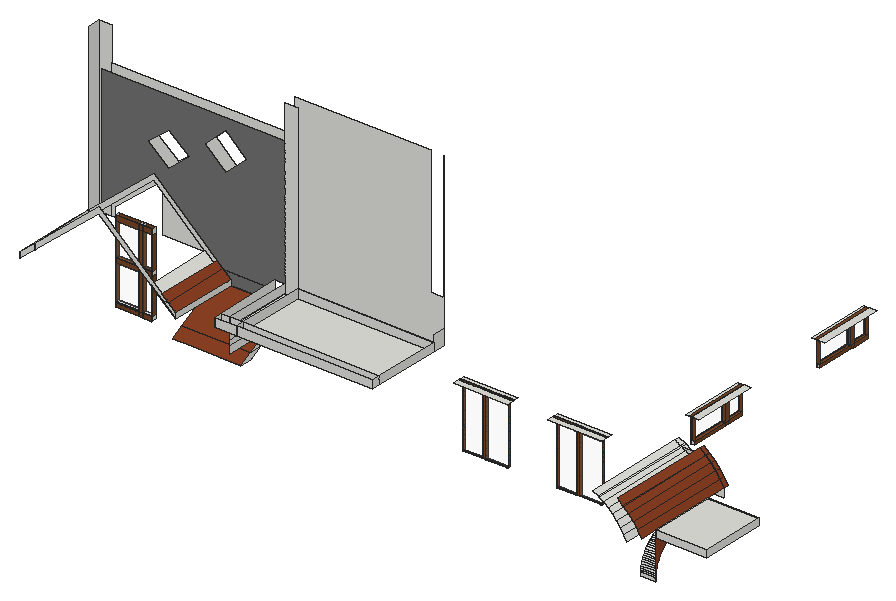
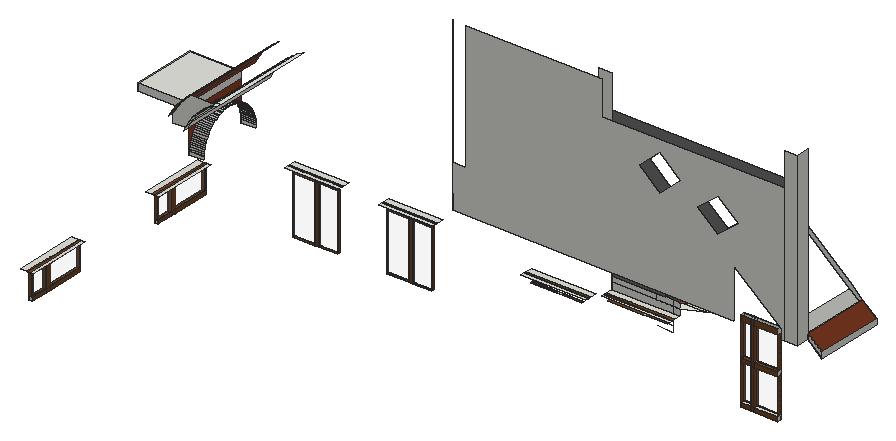
# SketchUp Ruby script. Lengths in inches.
U = 1.inch
M = Sketchup.active_model
def pt(a) = Geom::Point3d.new(a.map { |v| v * U })
def face(e, loops, mat)
  f = e.add_face(loops[0].map { |a| pt(a) })
  loops[1..].each { |l| e.add_face(l.map { |a| pt(a) }).erase! }
  f.material = f.back_material = mat if mat
  f
end
# faces: each face lists its corners as indices into pts; further lists are holes
def faces(e, pts, list, mat = nil) = list.each { |f| face(e, (f[0].is_a?(Array) ? f : [f]).map { |l| l.map { |i| pts[i] } }, mat) }
# xy, xz, yz: faces in a plane at the given z, y or x. An outline is a flat list of corners, or four numbers for a rectangle; further outlines are holes
def ring(l) = l.size == 4 ? [[l[0], l[1]], [l[2], l[1]], [l[2], l[3]], [l[0], l[3]]] : l.each_slice(2).to_a
def flat(e, list, mat, &to3) = list.each { |f| face(e, (f[0].is_a?(Array) ? f : [f]).map { |l| ring(l).map { |u, v| to3.(u, v) } }, mat) }
def xy(e, z, list, mat = nil) = flat(e, list, mat) { |x, y| [x, y, z] }
def xz(e, y, list, mat = nil) = flat(e, list, mat) { |x, z| [x, y, z] }
def yz(e, x, list, mat = nil) = flat(e, list, mat) { |y, z| [x, y, z] }
def lines(e, pts, list) = list.each { |a, b| e.add_line(pt(pts[a]), pt(pts[b])) }
# prism: a flat outline (further loops are holes) pulled along v
def prism(e, loops, v, mat = nil)
  f = face(e, loops, mat); d = Geom::Vector3d.new(v.map { |x| x * U })
  f.pushpull(f.normal.samedirection?(d) ? d.length : -d.length)
end
def box(e, o, s, mat = nil) = prism(e, [[o, [o[0] + s[0], o[1], o[2]], [o[0] + s[0], o[1] + s[1], o[2]], [o[0], o[1] + s[1], o[2]]]], [0, 0, s[2]], mat)
def at(x, y, z, deg = 0) = Geom::Transformation.translation(pt([x, y, z])) * Geom::Transformation.rotation(ORIGIN, Z_AXIS, deg.degrees)
def axes(o, x, y, z) = Geom::Transformation.new([*x, 0, *y, 0, *z, 0, *pt(o).to_a, 1])
def part(name) = M.definitions.add(name)
# library, detail: a bought-in or finely detailed component or shape, given as its bounding box
def library(name, o, s) = part(name).tap { |d| box(d.entities, o, s) }
def detail(e, o, s) = box(e.add_group.entities, o, s)
def put(e, d, t, mat = nil) = e.add_instance(d, t).tap { |i| i.material = mat if mat }
def group(e, t, mat = nil) = e.add_group.tap { |g| g.transformation = t; g.material = mat if mat }.entities
root = M.entities
M.materials.add("Glass Thin Clear 001").color = [243, 240, 240]
M.materials["Glass Thin Clear 001"].alpha = 0.1
M.materials.add("[Color M05]").color = [114, 114, 114]
M.materials.add("[Roofing Tile Spanish]").color = [138, 64, 36]
M.materials.add("[Wood Veneer 01]").color = [120, 70, 37]
xy(root,61.76,[[283.58,170.5625,285.96,172.1875],[349.83,170.5625,352.21,172.1875]])
xy(root,61.76,[[270.03,170.5625,283.58,170.875],[285.96,170.5625,301.89,170.875],[336.28,170.5625,349.83,170.875],[352.21,170.5625,368.14,170.875],[270.03,170.875,283.58,172.1875],
  [285.96,170.875,301.89,172.1875],[336.28,170.875,349.83,172.1875],[352.21,170.875,368.14,172.1875]],"[Wood Veneer 01]")
xy(root,66.22,[[41.61,170.5625,44.06,171.0625],[41.61,171.0625,44.06,173.875]])
xy(root,66.22,[[25.1,170.5625,41.61,171.0625],[44.06,170.5625,50.73,171.0625],[25.1,171.0625,41.61,173.875],[44.06,171.0625,50.73,173.875]],"[Wood Veneer 01]")
xy(root,69.18,[[41.61,170.5625,44.06,171.0625],[25.1,171.0625,41.61,173.875],[41.61,171.0625,44.06,173.875],[44.06,171.0625,50.73,173.875]])
xy(root,69.18,[[25.1,170.5625,41.61,171.0625],[44.06,170.5625,50.73,171.0625]],"[Wood Veneer 01]")
xy(root,91.5625,[[99.96,127.4375,99.96,135.72,113.85,135.72,113.21,127.4375],[113.21,127.4375,113.85,135.72,147.96,135.72,147.96,127.4375]])
xy(root,91.75,[[177.76,170.5625,182.03,172.375]])
xy(root,91.75,[[163.76,170.5625,177.76,170.875],[182.03,170.5625,200.3125,170.875],[163.76,170.875,177.76,172.375],[182.03,170.875,200.3125,172.375]],"[Wood Veneer 01]")
xy(root,93.98,[[399.27,210.14,401.46,237.2],[398.84,237.2,401.46,239.92],[399.27,239.92,401.46,252.12],[399.27,320.77,401.46,347.83],[398.84,347.83,401.46,350.54],
  [399.27,350.54,401.46,362.74]])
xy(root,93.98,[[398.84,210.14,399.27,237.2],[398.84,239.92,399.27,252.12],[398.84,320.77,399.27,347.83],[398.84,350.54,399.27,362.74]],"[Wood Veneer 01]")
xy(root,94.5,[[41.61,170.5625,44.06,171.0625],[41.61,171.0625,44.06,173.875]])
xy(root,94.5,[[25.1,170.5625,41.61,171.0625],[44.06,170.5625,50.73,171.0625],[25.1,171.0625,41.61,173.875],[44.06,171.0625,50.73,173.875]],"[Wood Veneer 01]")
xy(root,95.875,[[99.96,135.72,101.32,135.72,101.9375,143.8,99.96,143.8],[101.32,135.72,113.85,135.72,114.47,143.8,101.9375,143.8],[113.85,135.72,147.96,135.72,147.96,143.8,114.47,143.8]])
xy(root,96.1,[[159.41,166.0625,204.66,170.5625],[159.41,172.375,204.66,175.0625]])
xy(root,96.1,[[159.41,170.5625,204.66,171.8125],[159.41,171.8125,204.66,172.375]],"[Wood Veneer 01]")
xy(root,96.26,[[398.84,237.2,401.46,239.92],[398.84,347.83,401.46,350.54]])
xy(root,96.26,[[398.84,210.14,399.27,237.2],[399.27,210.14,401.46,237.2],[398.84,239.92,399.27,252.12],[399.27,239.92,401.46,252.12],[398.84,320.77,399.27,347.83],
  [399.27,320.77,401.46,347.83],[398.84,350.54,399.27,362.74],[399.27,350.54,401.46,362.74]],"[Wood Veneer 01]")
xy(root,97.27,[[25.1,170.5625,41.61,171.0625],[41.61,170.5625,44.06,171.0625],[44.06,170.5625,50.73,171.0625],[41.61,171.0625,44.06,173.875]])
xy(root,97.27,[[25.1,171.0625,41.61,173.875],[44.06,171.0625,50.73,173.875]],"[Wood Veneer 01]")
xy(root,100.14,[[117.68,170.5625,120.35,173.4375]])
xy(root,100.14,[[102.81,170.5625,117.68,171.125],[120.35,170.5625,145.12,171.125],[102.81,171.125,117.68,173.4375],[120.35,171.125,145.12,173.4375]],"[Wood Veneer 01]")
xy(root,100.61,[[457.27,105.875,493.27,151.74]])
xy(root,101.99,[[283.58,170.5625,285.96,172.1875],[349.83,170.5625,352.21,172.1875]])
xy(root,101.99,[[270.03,170.5625,283.58,170.875],[285.96,170.5625,301.89,170.875],[336.28,170.5625,349.83,170.875],[352.21,170.5625,368.14,170.875],[270.03,170.875,283.58,172.1875],
  [285.96,170.875,301.89,172.1875],[336.28,170.875,349.83,172.1875],[352.21,170.875,368.14,172.1875]],"[Wood Veneer 01]")
xy(root,102.98,[[99.96,166.0625,147.96,170.5625],[99.96,173.4375,147.96,175.0625]])
xy(root,102.98,[[99.96,170.5625,147.96,172.375],[99.96,172.375,147.96,173.4375]],"[Wood Veneer 01]")
xy(root,105.09,[[266.93,166.0625,304.99,170.5625],[333.18,166.0625,371.24,170.5625],[266.93,172.1875,304.99,175.0625],[333.18,172.1875,371.24,175.0625]])
xy(root,105.09,[[266.93,170.5625,304.99,171.8125],[333.18,170.5625,371.24,171.8125],[266.93,171.8125,304.99,172.1875],[333.18,171.8125,371.24,172.1875]],"[Wood Veneer 01]")
xy(root,105.64,[[457.27,105.875,493.27,151.74]])
xy(root,110.75,[[399.27,210.14,401.46,237.2],[398.84,237.2,401.46,239.92],[399.27,239.92,401.46,252.12],[399.27,320.77,401.46,347.83],[398.84,347.83,401.46,350.54],
  [399.27,350.54,401.46,362.74]])
xy(root,110.75,[[398.84,210.14,399.27,237.2],[398.84,239.92,399.27,252.12],[398.84,320.77,399.27,347.83],[398.84,350.54,399.27,362.74]],"[Wood Veneer 01]")
xy(root,112.57,[[396.96,208.32,398.84,253.94],[401.46,208.32,405.96,253.94],[396.96,318.94,398.84,364.57],[401.46,318.94,405.96,364.57]])
xy(root,112.57,[[398.84,208.32,400.59,253.94],[400.59,208.32,401.46,253.94],[398.84,318.94,400.59,364.57],[400.59,318.94,401.46,364.57]],"[Wood Veneer 01]")
xy(root,120,[[141.15,112.5625,156.96,118.0625],[156.96,112.5625,252.96,118.0625],[99.96,118.0625,99.96,166.0625,103.65,166.0625,100.75,128.39,104.53,128.1,104.53,118.0625],[141.15,118.0625,147.96,166.0625],[147.96,118.0625,156.96,166.0625],
  [156.96,118.0625,252.96,166.0625],[104.53,128.1,100.75,128.39,103.65,166.0625,104.53,166.0625],[103.65,166.0625,116.18,166.0625,103.72,167.02]])
xy(root,120.79,[[41.61,170.5625,44.06,171.0625],[41.61,171.0625,44.06,173.875]])
xy(root,120.79,[[25.1,170.5625,41.61,171.0625],[44.06,170.5625,50.73,171.0625],[25.1,171.0625,41.61,173.875],[44.06,171.0625,50.73,173.875]],"[Wood Veneer 01]")
xz(root,105.875,[[446.88,73.29,457.27,75.69],[457.27,100.61,493.27,105.64]])
xz(root,112.5625,[[141.15,120,156.96,126],[156.96,120,252.96,126]])
xz(root,118.0625,[[0,111.45,9.96,120,9.96,124,0,115.45],[109.72,111.45,109.72,115.45,104.53,120,99.96,120],[9.96,120,18.96,127.72,55.42,159,91.87,127.08,99.96,120,104.53,120,99.96,124,55.42,163,18.96,131.72,9.96,124],[141.15,120,147.96,126],[147.96,120,156.96,126],
  [156.96,120,252.96,126]])
xz(root,151.74,[[446.88,73.29,457.27,75.69],[446.88,75.69,457.27,75.78],[457.27,100.61,493.27,105.64]])
xz(root,166.0625,[[446.88,99.6875,457.27,99.6875,457.27,105.64,454.61,110.13,451.55,114.36,448.11,118.29,444.67,121.5625,427.48,121.5625,430.54,119.68,434.02,117.06,437.24,114.11,440.16,110.87,442.75,107.36,445,103.62],[99.96,102.98,147.96,107.76],[99.96,107.76,99.96,111.67,109.47,111.67,109.72,111.45,109.72,111.67,116.18,111.67,116.18,107.76],[116.18,107.76,147.96,111.67],[0,111.45,0,115.45,9.96,124,9.96,120],
  [109.72,111.45,109.47,111.67,109.72,111.67],[109.47,111.67,99.96,120,104.53,120,109.72,115.45,109.72,111.67],[9.96,120,9.96,124,18.96,131.72,55.42,163,99.96,124,104.53,120,99.96,120,91.87,127.08,55.42,159,18.96,127.72],[147.96,120,156.96,240],[156.96,120,252.96,126]])
xz(root,166.0625,[[99.96,111.67,109.47,111.67,99.96,120],[109.72,111.67,147.96,111.67,147.96,120,104.53,120,109.72,115.45],[[104.53,120,141.15,120,141.15,126,147.96,126,147.96,216.17,18.96,216.17,18.96,131.72,55.42,163,99.96,124],[106.65,181.57,91.87,195.01,106.65,208.45,121.43,195.01],[66.04,170.09,51.29,182.43,66.04,194.78,80.79,182.43]]],"[Color M05]")
xz(root,170.5625,[[283.58,61.76,285.96,101.99],[349.83,61.76,352.21,101.99],[25.1,66.22,41.61,69.18],[41.61,66.22,44.06,69.18],[44.06,66.22,50.73,69.18],
  [41.61,69.18,44.06,94.5],[25.1,94.5,41.61,97.27],[41.61,94.5,44.06,97.27],[44.06,94.5,50.73,97.27],[41.61,97.27,44.06,120.79],
  [25.1,120.79,41.61,124.49],[41.61,120.79,44.06,124.49],[44.06,120.79,50.73,124.49]],"[Wood Veneer 01]")
xz(root,170.875,[[270.03,61.76,283.58,101.99],[285.96,61.76,301.89,101.99],[336.28,61.76,349.83,101.99],[352.21,61.76,368.14,101.99]],"Glass Thin Clear 001")
xz(root,171.0625,[[25.1,66.22,41.61,69.18],[41.61,66.22,44.06,69.18],[44.06,66.22,50.73,69.18],[41.61,69.18,44.06,94.5],[25.1,94.5,41.61,97.27],
  [41.61,94.5,44.06,97.27],[44.06,94.5,50.73,97.27],[41.61,97.27,44.06,120.79],[25.1,120.79,41.61,124.49],[41.61,120.79,44.06,124.49],
  [44.06,120.79,50.73,124.49]])
xz(root,171.0625,[[25.1,69.18,41.61,94.5],[44.06,69.18,50.73,94.5],[25.1,97.27,41.61,120.79],[44.06,97.27,50.73,120.79]],"Glass Thin Clear 001")
xz(root,172.1875,[[283.58,61.76,285.96,101.99],[349.83,61.76,352.21,101.99]],"[Wood Veneer 01]")
xz(root,173.875,[[25.1,66.22,41.61,69.18],[41.61,66.22,44.06,69.18],[44.06,66.22,50.73,69.18],[41.61,69.18,44.06,94.5],[25.1,94.5,41.61,97.27],
  [41.61,94.5,44.06,97.27],[44.06,94.5,50.73,97.27],[41.61,97.27,44.06,120.79],[25.1,120.79,41.61,124.49],[41.61,120.79,44.06,124.49],
  [44.06,120.79,50.73,124.49]],"[Wood Veneer 01]")
xz(root,175.0625,[[9.96,120,18.96,240],[[18.96,120,18.96,216.17,147.96,216.17,147.96,240,243.5625,240,243.5625,150.4,252.8125,150.4,252.8125,240,252.96,240,252.96,120,54.79,120,54.79,154.64,21.04,126.39,21.04,120],[106.65,181.57,121.43,195.01,106.65,208.45,91.87,195.01],[66.04,170.09,80.79,182.43,66.04,194.78,51.29,182.43]]])
xz(root,210.14,[[398.84,93.98,401.46,96.26]])
xz(root,210.14,[[398.84,96.26,399.27,110.75],[399.27,96.26,401.46,110.75]],"[Wood Veneer 01]")
xz(root,237.2,[[398.84,93.98,401.46,96.26]])
xz(root,237.2,[[398.84,96.26,399.27,110.75],[399.27,96.26,401.46,110.75]],"[Wood Veneer 01]")
xz(root,239.92,[[398.84,93.98,401.46,96.26]])
xz(root,239.92,[[398.84,96.26,399.27,110.75],[399.27,96.26,401.46,110.75]],"[Wood Veneer 01]")
xz(root,252.12,[[398.84,93.98,401.46,96.26]])
xz(root,252.12,[[398.84,96.26,399.27,110.75],[399.27,96.26,401.46,110.75]],"[Wood Veneer 01]")
xz(root,320.77,[[398.84,93.98,401.46,96.26]])
xz(root,320.77,[[398.84,96.26,399.27,110.75],[399.27,96.26,401.46,110.75]],"[Wood Veneer 01]")
xz(root,347.83,[[398.84,93.98,401.46,96.26]])
xz(root,347.83,[[398.84,96.26,399.27,110.75],[399.27,96.26,401.46,110.75]],"[Wood Veneer 01]")
xz(root,350.54,[[398.84,93.98,401.46,96.26]])
xz(root,350.54,[[398.84,96.26,399.27,110.75],[399.27,96.26,401.46,110.75]],"[Wood Veneer 01]")
xz(root,362.74,[[398.84,93.98,401.46,96.26]])
xz(root,362.74,[[398.84,96.26,399.27,110.75],[399.27,96.26,401.46,110.75]],"[Wood Veneer 01]")
yz(root,0,[[118.0625,111.45,166.0625,115.45]])
yz(root,9.96,[[118.0625,120,166.0625,124],[166.0625,120,175.0625,240]])
yz(root,25.1,[[170.5625,66.22,171.0625,69.18],[171.0625,66.22,173.875,69.18],[170.5625,94.5,171.0625,97.27],[171.0625,94.5,173.875,97.27],[170.5625,120.79,171.0625,124.49],
  [171.0625,120.79,173.875,124.49]])
yz(root,25.1,[[170.5625,69.18,171.0625,94.5],[171.0625,69.18,173.875,94.5],[170.5625,97.27,171.0625,120.79],[171.0625,97.27,173.875,120.79]],"[Wood Veneer 01]")
yz(root,41.61,[[170.5625,66.22,171.0625,69.18],[171.0625,66.22,173.875,69.18],[170.5625,94.5,171.0625,97.27],[171.0625,94.5,173.875,97.27],[170.5625,120.79,171.0625,124.49],
  [171.0625,120.79,173.875,124.49]])
yz(root,41.61,[[170.5625,69.18,171.0625,94.5],[171.0625,69.18,173.875,94.5],[170.5625,97.27,171.0625,120.79],[171.0625,97.27,173.875,120.79]],"[Wood Veneer 01]")
yz(root,44.06,[[170.5625,66.22,171.0625,69.18],[171.0625,66.22,173.875,69.18],[170.5625,69.18,171.0625,94.5],[170.5625,94.5,171.0625,97.27],[171.0625,94.5,173.875,97.27],
  [170.5625,97.27,171.0625,120.79],[170.5625,120.79,171.0625,124.49],[171.0625,120.79,173.875,124.49]])
yz(root,44.06,[[171.0625,69.18,173.875,94.5],[171.0625,97.27,173.875,120.79]],"[Wood Veneer 01]")
yz(root,50.73,[[170.5625,66.22,171.0625,69.18],[171.0625,66.22,173.875,69.18],[170.5625,94.5,171.0625,97.27],[171.0625,94.5,173.875,97.27],[170.5625,120.79,171.0625,124.49],
  [171.0625,120.79,173.875,124.49]])
yz(root,50.73,[[170.5625,69.18,171.0625,94.5],[171.0625,69.18,173.875,94.5],[170.5625,97.27,171.0625,120.79],[171.0625,97.27,173.875,120.79]],"[Wood Veneer 01]")
yz(root,109.72,[[118.0625,111.45,166.0625,115.45]])
yz(root,141.15,[[112.5625,120,118.0625,126],[118.0625,120,166.0625,126]])
yz(root,147.96,[[127.4375,91.5625,135.72,91.5625,143.8,95.875,135.72,95.875],[127.4375,91.5625,135.72,95.875,143.8,95.875,135.72,91.5625],[135.72,95.875,149.375,102.98,157.11,102.98,143.8,95.875],[118.0625,102.98,118.0625,107.76,158.56,107.76,149.375,102.98],[149.375,102.98,157.11,102.98,166.0625,107.76,158.56,107.76],
  [157.11,102.98,166.0625,107.76,166.0625,102.98],[118.0625,107.76,118.0625,111.67,166.0625,111.67,158.56,107.76],[158.56,107.76,166.0625,107.76,166.0625,111.67],[118.0625,111.67,166.0625,120],[118.0625,120,166.0625,126]])
yz(root,156.96,[[112.5625,120,118.0625,126],[118.0625,120,166.0625,126]])
yz(root,252.96,[[112.5625,120,118.0625,126],[118.0625,120,166.0625,126],[166.0625,120,175.0625,130.625]])
yz(root,270.03,[[170.5625,61.76,170.875,101.99],[170.875,61.76,172.1875,101.99]],"[Wood Veneer 01]")
yz(root,283.58,[[170.5625,61.76,170.875,101.99],[170.875,61.76,172.1875,101.99]],"[Wood Veneer 01]")
yz(root,285.96,[[170.5625,61.76,170.875,101.99],[170.875,61.76,172.1875,101.99]],"[Wood Veneer 01]")
yz(root,301.89,[[170.5625,61.76,170.875,101.99],[170.875,61.76,172.1875,101.99]],"[Wood Veneer 01]")
yz(root,336.28,[[170.5625,61.76,170.875,101.99],[170.875,61.76,172.1875,101.99]],"[Wood Veneer 01]")
yz(root,349.83,[[170.5625,61.76,170.875,101.99],[170.875,61.76,172.1875,101.99]],"[Wood Veneer 01]")
yz(root,352.21,[[170.5625,61.76,170.875,101.99],[170.875,61.76,172.1875,101.99]],"[Wood Veneer 01]")
yz(root,368.14,[[170.5625,61.76,170.875,101.99],[170.875,61.76,172.1875,101.99]],"[Wood Veneer 01]")
yz(root,398.84,[[210.14,93.98,237.2,96.26],[237.2,93.98,239.92,96.26],[239.92,93.98,252.12,96.26],[320.77,93.98,347.83,96.26],[347.83,93.98,350.54,96.26],
  [350.54,93.98,362.74,96.26],[237.2,96.26,239.92,110.75],[347.83,96.26,350.54,110.75]],"[Wood Veneer 01]")
yz(root,399.27,[[210.14,96.26,237.2,110.75],[239.92,96.26,252.12,110.75],[320.77,96.26,347.83,110.75],[350.54,96.26,362.74,110.75]],"Glass Thin Clear 001")
yz(root,401.46,[[210.14,93.98,237.2,96.26],[237.2,93.98,239.92,96.26],[239.92,93.98,252.12,96.26],[320.77,93.98,347.83,96.26],[347.83,93.98,350.54,96.26],
  [350.54,93.98,362.74,96.26],[237.2,96.26,239.92,110.75],[347.83,96.26,350.54,110.75]],"[Wood Veneer 01]")
yz(root,457.27,[[105.875,73.29,105.875,75.69,105.84,74.54],[151.74,73.29,151.78,74.54,151.74,75.69],[105.875,100.61,151.74,105.64]])
yz(root,457.27,[[105.875,73.29,105.84,74.54,105.875,75.69,105.88,75.78,105.98,77.02,106.15,78.25,106.38,79.47,106.68,80.68,107.05,81.86,107.48,83.03,107.97,84.17,108.53,85.29,109.14,86.37,109.81,87.41,110.53,88.42,111.3125,89.39,112.14,90.32,113.02,91.2,113.95,92.02,114.92,92.8,115.93,93.53,116.98,94.2,118.06,94.81,119.17,95.36,120.3125,95.85,121.48,96.28,122.67,96.64,123.875,96.94,125.1,97.18,126.33,97.35,127.57,97.45,128.81,97.48,130.05,97.45,131.29,97.35,132.52,97.18,133.74,96.94,134.95,96.64,136.14,96.28,137.31,95.85,138.45,95.36,139.5625,94.81,140.64,94.2,141.69,93.53,142.7,92.8,143.67,92.02,144.6,91.2,145.48,90.32,146.31,89.39,147.09,88.42,147.8125,87.41,148.48,86.37,149.09,85.29,149.65,84.17,150.14,83.03,150.57,81.86,150.93,80.68,151.24,79.47,151.47,78.25,151.64,77.02,151.74,75.78,151.74,75.69,151.78,74.54,151.74,73.29,151.74,100.61,105.875,100.61]],"[Roofing Tile Spanish]")
yz(root,493.27,[[105.875,100.61,151.74,105.64]])
p = [[457.27,105.88,75.78],[457.27,105.875,75.69],[446.88,105.875,75.69],[446.88,105.88,75.78],[457.27,105.98,77.02],[446.88,105.98,77.02],
  [457.27,151.74,75.78],[457.27,151.64,77.02],[446.88,151.64,77.02],[446.88,151.74,75.78],[457.27,106.15,78.25],[446.88,106.15,78.25],
  [457.27,151.47,78.25],[446.88,151.47,78.25],[457.27,106.38,79.47],[446.88,106.38,79.47],[457.27,151.24,79.47],[446.88,151.24,79.47],
  [457.27,106.68,80.68],[446.88,106.68,80.68],[457.27,150.93,80.68],[446.88,150.93,80.68],[457.27,107.05,81.86],[446.88,107.05,81.86],
  [457.27,150.57,81.86],[446.88,150.57,81.86],[457.27,107.48,83.03],[446.88,107.48,83.03],[457.27,150.14,83.03],[446.88,150.14,83.03],
  [457.27,107.97,84.17],[446.88,107.97,84.17],[457.27,149.65,84.17],[446.88,149.65,84.17],[457.27,108.53,85.29],[446.88,108.53,85.29],
  [457.27,149.09,85.29],[446.88,149.09,85.29],[457.27,109.14,86.37],[446.88,109.14,86.37],[457.27,148.48,86.37],[446.88,148.48,86.37],
  [457.27,109.81,87.41],[446.88,109.81,87.41],[457.27,147.8125,87.41],[446.88,147.8125,87.41],[457.27,110.53,88.42],[446.88,110.53,88.42],
  [457.27,147.09,88.42],[446.88,147.09,88.42],[457.27,111.3125,89.39],[446.88,111.3125,89.39],[457.27,146.31,89.39],[446.88,146.31,89.39],
  [457.27,112.14,90.32],[446.88,112.14,90.32],[457.27,145.48,90.32],[446.88,145.48,90.32],[457.27,113.02,91.2],[446.88,113.02,91.2],
  [457.27,144.6,91.2],[446.88,144.6,91.2],[457.27,113.95,92.02],[446.88,113.95,92.02],[457.27,143.67,92.02],[446.88,143.67,92.02],
  [147.96,127.4375,91.5625],[147.96,135.72,95.875],[113.85,135.72,95.875],[101.32,135.72,95.875],[99.96,135.72,95.875],[99.96,127.4375,91.5625],
  [113.21,127.4375,91.5625],[147.96,143.8,95.875],[147.96,135.72,91.5625],[113.85,135.72,91.5625],[99.96,135.72,91.5625],[99.96,143.8,95.875],
  [101.9375,143.8,95.875],[114.47,143.8,95.875],[457.27,114.92,92.8],[446.88,114.92,92.8],[457.27,142.7,92.8],[446.88,142.7,92.8],
  [457.27,115.93,93.53],[446.88,115.93,93.53],[457.27,141.69,93.53],[446.88,141.69,93.53],[457.27,116.98,94.2],[446.88,116.98,94.2],
  [457.27,140.64,94.2],[446.88,140.64,94.2],[457.27,118.06,94.81],[446.88,118.06,94.81],[457.27,139.5625,94.81],[446.88,139.5625,94.81],
  [457.27,119.17,95.36],[446.88,119.17,95.36],[457.27,138.45,95.36],[446.88,138.45,95.36],[457.27,120.3125,95.85],[446.88,120.3125,95.85],
  [457.27,137.31,95.85],[446.88,137.31,95.85],[457.27,121.48,96.28],[446.88,121.48,96.28],[147.96,158.56,107.76],[147.96,166.0625,111.67],
  [116.18,166.0625,111.67],[109.72,166.0625,111.67],[109.47,166.0625,111.67],[99.96,166.0625,111.67],[147.96,149.375,102.98],[457.27,136.14,96.28],
  [446.88,136.14,96.28],[147.96,166.0625,107.76],[147.96,157.11,102.98],[99.96,166.0625,107.76],[116.18,166.0625,107.76],[457.27,122.67,96.64],
  [446.88,122.67,96.64],[457.27,134.95,96.64],[446.88,134.95,96.64],[457.27,123.875,96.94],[446.88,123.875,96.94],[457.27,133.74,96.94],
  [446.88,133.74,96.94],[457.27,125.1,97.18],[446.88,125.1,97.18],[457.27,132.52,97.18],[446.88,132.52,97.18],[457.27,126.33,97.35],
  [446.88,126.33,97.35],[457.27,131.29,97.35],[446.88,131.29,97.35],[457.27,127.57,97.45],[446.88,127.57,97.45],[457.27,130.05,97.45],
  [446.88,130.05,97.45],[457.27,128.81,97.48],[446.88,128.81,97.48],[445,93.6875,103.62],[445,166.0625,103.62],[446.88,166.0625,99.6875],
  [446.88,93.6875,99.6875],[445,169.5,103.62],[446.88,169.5,99.6875],[442.75,93.6875,107.36],[442.75,166.0625,107.36],[442.75,169.5,107.36],
  [457.27,151.74,105.64],[457.27,166.0625,105.64],[454.61,166.0625,110.13],[454.61,93.6875,110.13],[457.27,93.6875,105.64],[457.27,105.875,105.64],
  [457.27,169.5,105.64],[454.61,169.5,110.13],[440.16,93.6875,110.87],[440.16,166.0625,110.87],[440.16,169.5,110.87],[451.55,166.0625,114.36],
  [451.55,93.6875,114.36],[451.55,169.5,114.36],[437.24,93.6875,114.11],[437.24,166.0625,114.11],[437.24,169.5,114.11],[0,166.0625,111.45],
  [9.96,166.0625,120],[9.96,118.0625,120],[0,118.0625,111.45],[99.96,166.0625,120],[109.72,166.0625,111.45],[109.72,118.0625,111.45],
  [99.96,118.0625,120],[434.02,93.6875,117.06],[434.02,166.0625,117.06],[434.02,169.5,117.06],[448.11,166.0625,118.29],[448.11,93.6875,118.29],
  [448.11,169.5,118.29],[9.96,166.0625,124],[0,166.0625,115.45],[0,118.0625,115.45],[9.96,118.0625,124],[109.72,166.0625,115.45],
  [104.53,166.0625,120],[104.53,128.1,120],[104.53,118.0625,120],[109.72,118.0625,115.45],[430.54,93.6875,119.68],[430.54,166.0625,119.68],
  [430.54,169.5,119.68],[444.67,166.0625,121.5625],[444.67,93.6875,121.5625],[444.67,169.5,121.5625],[427.48,93.6875,121.5625],[427.48,166.0625,121.5625],
  [427.48,169.5,121.5625],[18.96,166.0625,127.72],[18.96,118.0625,127.72],[91.87,166.0625,127.08],[91.87,118.0625,127.08],[99.96,166.0625,124],
  [99.96,118.0625,124],[426.82,93.6875,121.97],[426.82,166.0625,121.97],[444.33,166.0625,121.88],[444.33,93.6875,121.88],[426.82,169.5,121.97],
  [444.33,169.5,121.88],[440.24,166.0625,125.125],[440.24,93.6875,125.125],[440.24,169.5,125.125],[422.91,93.6875,123.88],[422.91,166.0625,123.88],
  [422.91,169.5,123.88],[103.72,167.02,120],[103.72,167.02,95.875],[116.18,166.0625,95.875],[116.18,166.0625,91.5625],[103.72,167.02,91.5625]]
faces(root,p,[[0,1,2,3],[4,0,3,5],[6,7,8,9],[10,4,5,11],[7,12,13,8],[14,10,11,15],[12,16,17,13],[18,14,15,19],
  [16,20,21,17],[22,18,19,23],[20,24,25,21],[26,22,23,27],[24,28,29,25],[30,26,27,31],[28,32,33,29],[34,30,31,35],
  [32,36,37,33],[38,34,35,39],[36,40,41,37],[42,38,39,43],[40,44,45,41],[46,42,43,47],[44,48,49,45],[50,46,47,51],
  [48,52,53,49],[54,50,51,55],[52,56,57,53],[58,54,55,59],[56,60,61,57],[62,58,59,63],[60,64,65,61],[73,74,75,76,77,78,79],
  [80,62,63,81],[64,82,83,65],[84,80,81,85],[82,86,87,83],[88,84,85,89],[86,90,91,87],[92,88,89,93],[90,94,95,91],
  [96,92,93,97],[94,98,99,95],[100,96,97,101],[98,102,103,99],[104,100,101,105],[102,113,114,103],[115,116,73,79,78,77,117,118],[119,104,105,120],
  [113,121,122,114],[123,119,120,124],[121,125,126,122],[127,123,124,128],[125,129,130,126],[131,127,128,132],[129,133,134,130],[135,131,132,136],
  [133,137,138,134],[139,135,136,140],[137,139,140,138],[141,142,143,144],[143,142,145,146],[147,148,142,141],[142,148,149,145],[158,159,148,147],
  [148,159,160,149],[164,165,159,158],[159,165,166,160],[167,168,169,170],[171,110,172,173,174],[175,176,165,164],[165,176,177,166],[190,191,176,175],
  [176,191,192,177],[196,197,191,190],[191,197,198,192],[168,199,200,169],[201,171,174,202],[205,206,197,196],[197,206,209,198],[214,215,206,205],
  [206,215,216,209]])
faces(root,p,[[66,67,68,69,70,71,72],[106,107,108,109,110,111,70,69,68,67,112],[150,151,152,153,154,155],[152,151,156,157],[153,152,161,162],[161,152,157,163],[162,161,178,179],[178,161,163,180],
  [181,182,183,184],[185,186,187,188,189],[179,178,193,194],[193,178,180,195],[186,203,204,188,187],[194,193,207,208],[207,193,195,210],[208,207,211,212],
  [211,207,210,213]],"[Roofing Tile Spanish]")
lines(root,p,[[217,218],[219,218],[220,221],[218,221]])
